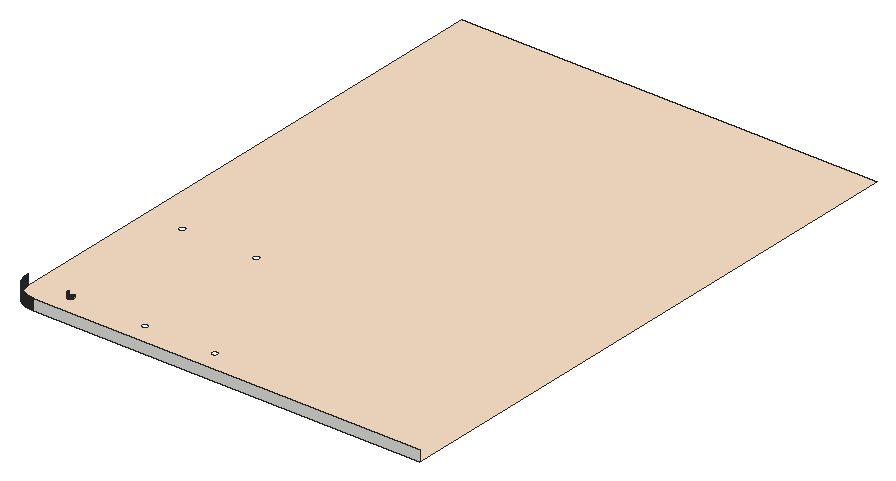
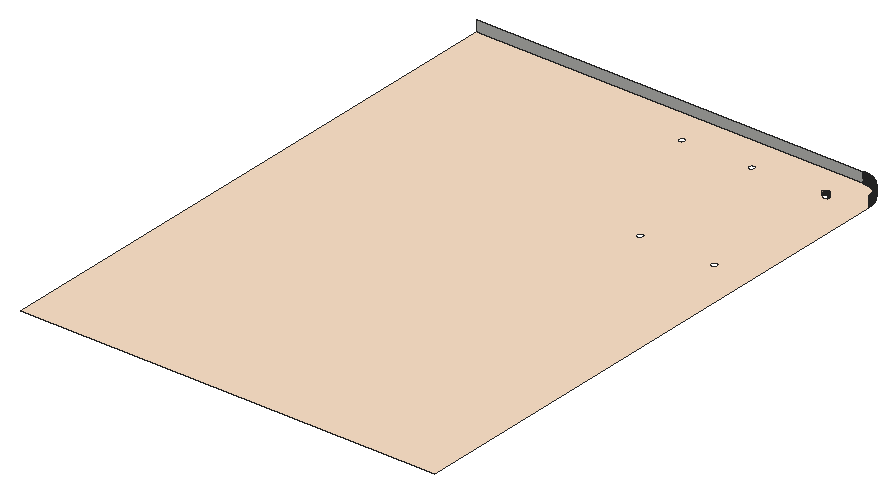
# SketchUp Ruby script. Lengths in inches.
U = 1.inch
M = Sketchup.active_model
def pt(a) = Geom::Point3d.new(a.map { |v| v * U })
def face(e, loops, mat)
  f = e.add_face(loops[0].map { |a| pt(a) })
  loops[1..].each { |l| e.add_face(l.map { |a| pt(a) }).erase! }
  f.material = f.back_material = mat if mat
  f
end
# faces: each face lists its corners as indices into pts; further lists are holes
def faces(e, pts, list, mat = nil) = list.each { |f| face(e, (f[0].is_a?(Array) ? f : [f]).map { |l| l.map { |i| pts[i] } }, mat) }
# xy, xz, yz: faces in a plane at the given z, y or x. An outline is a flat list of corners, or four numbers for a rectangle; further outlines are holes
def ring(l) = l.size == 4 ? [[l[0], l[1]], [l[2], l[1]], [l[2], l[3]], [l[0], l[3]]] : l.each_slice(2).to_a
def flat(e, list, mat, &to3) = list.each { |f| face(e, (f[0].is_a?(Array) ? f : [f]).map { |l| ring(l).map { |u, v| to3.(u, v) } }, mat) }
def xy(e, z, list, mat = nil) = flat(e, list, mat) { |x, y| [x, y, z] }
def xz(e, y, list, mat = nil) = flat(e, list, mat) { |x, z| [x, y, z] }
def yz(e, x, list, mat = nil) = flat(e, list, mat) { |y, z| [x, y, z] }
def lines(e, pts, list) = list.each { |a, b| e.add_line(pt(pts[a]), pt(pts[b])) }
# prism: a flat outline (further loops are holes) pulled along v
def prism(e, loops, v, mat = nil)
  f = face(e, loops, mat); d = Geom::Vector3d.new(v.map { |x| x * U })
  f.pushpull(f.normal.samedirection?(d) ? d.length : -d.length)
end
def box(e, o, s, mat = nil) = prism(e, [[o, [o[0] + s[0], o[1], o[2]], [o[0] + s[0], o[1] + s[1], o[2]], [o[0], o[1] + s[1], o[2]]]], [0, 0, s[2]], mat)
def at(x, y, z, deg = 0) = Geom::Transformation.translation(pt([x, y, z])) * Geom::Transformation.rotation(ORIGIN, Z_AXIS, deg.degrees)
def axes(o, x, y, z) = Geom::Transformation.new([*x, 0, *y, 0, *z, 0, *pt(o).to_a, 1])
def part(name) = M.definitions.add(name)
# library, detail: a bought-in or finely detailed component or shape, given as its bounding box
def library(name, o, s) = part(name).tap { |d| box(d.entities, o, s) }
def detail(e, o, s) = box(e.add_group.entities, o, s)
def put(e, d, t, mat = nil) = e.add_instance(d, t).tap { |i| i.material = mat if mat }
def group(e, t, mat = nil) = e.add_group.tap { |g| g.transformation = t; g.material = mat if mat }.entities
root = M.entities
M.materials.add("1122 AP 7994 PEACH ROSE").color = [254, 227, 201]
xy(root,149.82,[[[32.75,153,32.5,153.01,32.25,153.01,31.99,153.02,31.74,153.03,31.49,153.05,31.24,153.0625,30.99,153.08,30.74,153.11,30.49,153.13,30.24,153.16,29.99,153.1875,29.74,153.22,29.49,153.26,29.25,153.3,28.75,153.38,28.5,153.43,28.26,153.47,28.01,153.52,27.76,153.58,27.52,153.63,27.28,153.69,27.03,153.75,26.79,153.82,26.55,153.88,26.3,153.95,26.0625,154.02,25.82,154.1,25.58,154.17,25.34,154.25,25.11,154.33,24.63,154.51,24.4,154.59,24.17,154.69,23.93,154.78,23.47,154.97,23.24,155.07,23.01,155.18,22.78,155.28,22.55,155.39,22.33,155.5,22.1,155.62,21.88,155.73,21.66,155.85,21.4375,155.97,21.22,156.09,21,156.22,20.78,156.34,20.57,156.47,20.35,156.6,20.14,156.74,19.93,156.87,19.3,157.29,19.1,157.4375,18.89,157.58,18.49,157.88,18.29,158.04,18.09,158.19,17.9,158.35,17.7,158.51,17.32,158.83,17.13,159,16.94,159.16,16.75,159.33,16.57,159.5,16.39,159.68,16.21,159.85,15.85,160.21,15.68,160.39,15.5,160.57,15.33,160.75,15.16,160.94,15,161.13,14.83,161.32,14.51,161.7,14.35,161.9,14.19,162.09,14.04,162.29,13.88,162.49,13.58,162.89,13.4375,163.1,13.29,163.3,12.87,163.93,12.74,164.14,12.6,164.35,12.47,164.57,12.34,164.78,12.22,165,12.09,165.22,11.97,165.4375,11.85,165.66,11.73,165.88,11.62,166.1,11.5,166.33,11.39,166.55,11.28,166.78,11.18,167.01,11.07,167.24,10.97,167.47,10.78,167.93,10.69,168.17,10.59,168.4,10.51,168.63,10.33,169.11,10.25,169.34,10.17,169.58,10.1,169.82,10.02,170.0625,9.95,170.3,9.88,170.55,9.82,170.79,9.75,171.03,9.69,171.28,9.63,171.52,9.58,171.76,9.52,172.01,9.47,172.26,9.43,172.5,9.38,172.75,9.3,173.25,9.26,173.49,9.22,173.74,9.1875,173.99,9.16,174.24,9.13,174.49,9.11,174.74,9.08,174.99,9.0625,175.24,9.05,175.49,9.03,175.74,9.02,175.99,9.01,176.25,9.01,176.5,9,176.75,9,645,366,645,366,153],[40.86,180.07,41.17,180.07,41.49,180.11,41.5625,180.12,41.64,180.14,41.72,180.15,41.79,180.17,41.87,180.19,41.94,180.22,42.02,180.24,42.16,180.3,42.24,180.33,42.31,180.36,42.38,180.4,42.45,180.43,42.52,180.47,42.58,180.51,42.65,180.55,42.72,180.6,42.78,180.64,43.08,180.89,43.14,180.95,43.19,181.01,43.25,181.0625,43.3,181.12,43.4,181.24,43.44,181.31,43.49,181.37,43.53,181.4375,43.57,181.5,43.65,181.64,43.6875,181.71,43.72,181.78,43.76,181.85,43.79,181.92,43.82,182,43.84,182.07,43.87,182.14,43.89,182.22,43.91,182.29,43.95,182.45,43.97,182.52,44.01,182.84,44.01,182.91,44.02,182.99,44.02,183.15,44.01,183.23,44.01,183.31,44,183.38,43.97,183.62,43.95,183.69,43.91,183.85,43.89,183.92,43.87,184,43.84,184.07,43.82,184.15,43.76,184.29,43.72,184.36,43.6875,184.43,43.65,184.5,43.57,184.64,43.53,184.7,43.49,184.77,43.44,184.83,43.4,184.9,43.25,185.08,43.08,185.25,42.78,185.5,42.72,185.54,42.65,185.59,42.58,185.63,42.52,185.67,42.45,185.71,42.38,185.74,42.31,185.78,42.24,185.8125,42.16,185.84,42.02,185.9,41.94,185.92,41.87,185.95,41.79,185.97,41.72,185.99,41.64,186.01,41.5625,186.02,41.49,186.03,41.41,186.05,41.33,186.05,41.25,186.0625,41.17,186.07,40.86,186.07,40.78,186.0625,40.7,186.05,40.625,186.05,40.55,186.03,40.39,186.01,40.32,185.99,40.16,185.95,40.09,185.92,40.01,185.9,39.87,185.84,39.8,185.8125,39.72,185.78,39.65,185.74,39.58,185.71,39.52,185.67,39.38,185.59,39.32,185.54,39.25,185.5,38.95,185.25,38.84,185.14,38.74,185.02,38.68,184.96,38.64,184.9,38.59,184.83,38.54,184.77,38.5,184.7,38.46,184.64,38.34,184.43,38.28,184.29,38.24,184.22,38.22,184.15,38.1875,184.07,38.16,184,38.14,183.92,38.12,183.85,38.08,183.69,38.07,183.62,38.05,183.54,38.03,183.38,38.03,183.31,38.02,183.23,38.02,182.91,38.03,182.84,38.03,182.76,38.05,182.6,38.07,182.52,38.08,182.45,38.12,182.29,38.14,182.22,38.16,182.14,38.1875,182.07,38.22,182,38.24,181.92,38.28,181.85,38.34,181.71,38.46,181.5,38.5,181.4375,38.54,181.37,38.59,181.31,38.64,181.24,38.68,181.18,38.74,181.12,38.79,181.0625,38.84,181.01,38.89,180.95,38.95,180.89,39.25,180.64,39.32,180.6,39.38,180.55,39.52,180.47,39.58,180.43,39.65,180.4,39.72,180.36,39.8,180.33,40.01,180.24,40.09,180.22,40.16,180.19,40.32,180.15,40.39,180.14,40.47,180.12,40.55,180.11,40.7,180.09],[104.79,180.07,105.11,180.07,105.1875,180.08,105.26,180.09,105.5,180.12,105.57,180.14,105.65,180.15,105.73,180.17,105.8,180.19,105.88,180.22,105.95,180.24,106.03,180.27,106.24,180.36,106.3125,180.4,106.38,180.43,106.59,180.55,106.65,180.6,106.71,180.64,106.78,180.69,107.02,180.89,107.07,180.95,107.13,181.01,107.18,181.0625,107.23,181.12,107.33,181.24,107.38,181.31,107.42,181.37,107.47,181.4375,107.51,181.5,107.59,181.64,107.66,181.78,107.72,181.92,107.75,182,107.78,182.07,107.8,182.14,107.83,182.22,107.85,182.29,107.89,182.45,107.9,182.52,107.91,182.6,107.93,182.68,107.93,182.76,107.94,182.84,107.95,182.91,107.95,183.23,107.94,183.31,107.93,183.38,107.93,183.46,107.91,183.54,107.9,183.62,107.89,183.69,107.85,183.85,107.83,183.92,107.8,184,107.78,184.07,107.75,184.15,107.66,184.36,107.59,184.5,107.51,184.64,107.47,184.7,107.42,184.77,107.38,184.83,107.33,184.9,107.13,185.14,107.07,185.19,107.02,185.25,106.78,185.45,106.71,185.5,106.65,185.54,106.59,185.59,106.38,185.71,106.3125,185.74,106.24,185.78,106.17,185.8125,106.1,185.84,106.03,185.87,105.95,185.9,105.88,185.92,105.8,185.95,105.73,185.97,105.57,186.01,105.5,186.02,105.42,186.03,105.34,186.05,105.26,186.05,105.1875,186.0625,105.11,186.07,104.79,186.07,104.72,186.0625,104.64,186.05,104.56,186.05,104.48,186.03,104.4,186.02,104.33,186.01,104.17,185.97,104.1,185.95,104.02,185.92,103.95,185.9,103.8,185.84,103.73,185.8125,103.66,185.78,103.59,185.74,103.52,185.71,103.38,185.63,103.32,185.59,103.25,185.54,103.1875,185.5,103,185.35,102.94,185.3,102.72,185.08,102.57,184.9,102.52,184.83,102.48,184.77,102.44,184.7,102.39,184.64,102.31,184.5,102.28,184.43,102.24,184.36,102.15,184.15,102.125,184.07,102.1,184,102.07,183.92,102.05,183.85,102.03,183.77,102.02,183.69,102,183.62,101.97,183.38,101.96,183.31,101.96,183.23,101.95,183.15,101.95,182.99,101.96,182.91,101.96,182.84,102,182.52,102.02,182.45,102.03,182.37,102.05,182.29,102.07,182.22,102.1,182.14,102.15,182,102.18,181.92,102.24,181.78,102.28,181.71,102.31,181.64,102.39,181.5,102.44,181.4375,102.48,181.37,102.52,181.31,102.57,181.24,102.67,181.12,102.72,181.0625,102.78,181.01,102.83,180.95,102.94,180.84,103,180.79,103.1875,180.64,103.25,180.6,103.32,180.55,103.38,180.51,103.52,180.43,103.59,180.4,103.66,180.36,103.8,180.3,103.95,180.24,104.02,180.22,104.1,180.19,104.17,180.17,104.25,180.15,104.33,180.14,104.4,180.12,104.72,180.08],[164.79,180.07,165.11,180.07,165.1875,180.08,165.26,180.09,165.5,180.12,165.57,180.14,165.65,180.15,165.73,180.17,165.8,180.19,165.88,180.22,165.95,180.24,166.03,180.27,166.24,180.36,166.3125,180.4,166.38,180.43,166.59,180.55,166.65,180.6,166.71,180.64,166.78,180.69,167.02,180.89,167.07,180.95,167.13,181.01,167.18,181.0625,167.23,181.12,167.33,181.24,167.38,181.31,167.42,181.37,167.47,181.4375,167.51,181.5,167.59,181.64,167.66,181.78,167.72,181.92,167.75,182,167.78,182.07,167.8,182.14,167.83,182.22,167.85,182.29,167.89,182.45,167.9,182.52,167.91,182.6,167.93,182.68,167.93,182.76,167.94,182.84,167.95,182.91,167.95,183.23,167.94,183.31,167.93,183.38,167.93,183.46,167.91,183.54,167.9,183.62,167.89,183.69,167.85,183.85,167.83,183.92,167.8,184,167.78,184.07,167.75,184.15,167.66,184.36,167.59,184.5,167.51,184.64,167.47,184.7,167.42,184.77,167.38,184.83,167.33,184.9,167.13,185.14,167.07,185.19,167.02,185.25,166.78,185.45,166.71,185.5,166.65,185.54,166.59,185.59,166.38,185.71,166.3125,185.74,166.24,185.78,166.17,185.8125,166.1,185.84,166.03,185.87,165.95,185.9,165.88,185.92,165.8,185.95,165.73,185.97,165.57,186.01,165.5,186.02,165.42,186.03,165.34,186.05,165.26,186.05,165.1875,186.0625,165.11,186.07,164.79,186.07,164.72,186.0625,164.64,186.05,164.56,186.05,164.48,186.03,164.4,186.02,164.33,186.01,164.17,185.97,164.1,185.95,164.02,185.92,163.95,185.9,163.8,185.84,163.73,185.8125,163.66,185.78,163.59,185.74,163.52,185.71,163.38,185.63,163.32,185.59,163.25,185.54,163.1875,185.5,163,185.35,162.94,185.3,162.72,185.08,162.57,184.9,162.52,184.83,162.48,184.77,162.44,184.7,162.39,184.64,162.31,184.5,162.28,184.43,162.24,184.36,162.15,184.15,162.125,184.07,162.1,184,162.07,183.92,162.05,183.85,162.03,183.77,162.02,183.69,162,183.62,161.97,183.38,161.96,183.31,161.96,183.23,161.95,183.15,161.95,182.99,161.96,182.91,161.96,182.84,162,182.52,162.02,182.45,162.03,182.37,162.05,182.29,162.07,182.22,162.1,182.14,162.15,182,162.18,181.92,162.24,181.78,162.28,181.71,162.31,181.64,162.39,181.5,162.44,181.4375,162.48,181.37,162.52,181.31,162.57,181.24,162.67,181.12,162.72,181.0625,162.78,181.01,162.83,180.95,162.94,180.84,163,180.79,163.1875,180.64,163.25,180.6,163.32,180.55,163.38,180.51,163.52,180.43,163.59,180.4,163.66,180.36,163.8,180.3,163.95,180.24,164.02,180.22,164.1,180.19,164.17,180.17,164.25,180.15,164.33,180.14,164.4,180.12,164.72,180.08],[104.79,300.07,105.11,300.07,105.1875,300.08,105.26,300.09,105.5,300.12,105.57,300.14,105.65,300.15,105.73,300.17,105.8,300.19,105.88,300.22,105.95,300.24,106.03,300.27,106.24,300.36,106.3125,300.4,106.38,300.43,106.59,300.55,106.65,300.6,106.71,300.64,106.78,300.69,107.02,300.89,107.07,300.95,107.13,301.01,107.18,301.0625,107.23,301.12,107.33,301.24,107.38,301.31,107.42,301.37,107.47,301.4375,107.51,301.5,107.59,301.64,107.66,301.78,107.72,301.92,107.75,302,107.78,302.07,107.8,302.14,107.83,302.22,107.85,302.29,107.89,302.45,107.9,302.52,107.91,302.6,107.93,302.68,107.93,302.76,107.94,302.84,107.95,302.91,107.95,303.23,107.94,303.31,107.93,303.38,107.93,303.46,107.91,303.54,107.9,303.62,107.89,303.69,107.85,303.85,107.83,303.92,107.8,304,107.78,304.07,107.75,304.15,107.66,304.36,107.59,304.5,107.51,304.64,107.47,304.7,107.42,304.77,107.38,304.83,107.33,304.9,107.13,305.14,107.07,305.19,107.02,305.25,106.78,305.45,106.71,305.5,106.65,305.54,106.59,305.59,106.38,305.71,106.3125,305.74,106.24,305.78,106.17,305.8125,106.1,305.84,106.03,305.87,105.95,305.9,105.88,305.92,105.8,305.95,105.73,305.97,105.57,306.01,105.5,306.02,105.42,306.03,105.34,306.05,105.26,306.05,105.1875,306.0625,105.11,306.07,104.79,306.07,104.72,306.0625,104.64,306.05,104.56,306.05,104.48,306.03,104.4,306.02,104.33,306.01,104.17,305.97,104.1,305.95,104.02,305.92,103.95,305.9,103.8,305.84,103.73,305.8125,103.66,305.78,103.59,305.74,103.52,305.71,103.38,305.63,103.32,305.59,103.25,305.54,103.1875,305.5,103,305.35,102.94,305.3,102.72,305.08,102.57,304.9,102.52,304.83,102.48,304.77,102.44,304.7,102.39,304.64,102.31,304.5,102.28,304.43,102.24,304.36,102.15,304.15,102.125,304.07,102.1,304,102.07,303.92,102.05,303.85,102.03,303.77,102.02,303.69,102,303.62,101.97,303.38,101.96,303.31,101.96,303.23,101.95,303.15,101.95,302.99,101.96,302.91,101.96,302.84,102,302.52,102.02,302.45,102.03,302.37,102.05,302.29,102.07,302.22,102.1,302.14,102.15,302,102.18,301.92,102.24,301.78,102.28,301.71,102.31,301.64,102.39,301.5,102.44,301.4375,102.48,301.37,102.52,301.31,102.57,301.24,102.67,301.12,102.72,301.0625,102.78,301.01,102.83,300.95,102.94,300.84,103,300.79,103.1875,300.64,103.25,300.6,103.32,300.55,103.38,300.51,103.52,300.43,103.59,300.4,103.66,300.36,103.8,300.3,103.95,300.24,104.02,300.22,104.1,300.19,104.17,300.17,104.25,300.15,104.33,300.14,104.4,300.12,104.72,300.08],[40.86,300.07,41.17,300.07,41.49,300.11,41.5625,300.12,41.64,300.14,41.72,300.15,41.79,300.17,41.87,300.19,41.94,300.22,42.02,300.24,42.16,300.3,42.24,300.33,42.31,300.36,42.38,300.4,42.45,300.43,42.52,300.47,42.58,300.51,42.65,300.55,42.72,300.6,42.78,300.64,43.08,300.89,43.14,300.95,43.19,301.01,43.25,301.0625,43.3,301.12,43.4,301.24,43.44,301.31,43.49,301.37,43.53,301.4375,43.57,301.5,43.65,301.64,43.6875,301.71,43.72,301.78,43.76,301.85,43.79,301.92,43.82,302,43.84,302.07,43.87,302.14,43.89,302.22,43.91,302.29,43.95,302.45,43.97,302.52,44.01,302.84,44.01,302.91,44.02,302.99,44.02,303.15,44.01,303.23,44.01,303.31,44,303.38,43.97,303.62,43.95,303.69,43.91,303.85,43.89,303.92,43.87,304,43.84,304.07,43.82,304.15,43.76,304.29,43.72,304.36,43.6875,304.43,43.65,304.5,43.57,304.64,43.53,304.7,43.49,304.77,43.44,304.83,43.4,304.9,43.25,305.08,43.08,305.25,42.78,305.5,42.72,305.54,42.65,305.59,42.58,305.63,42.52,305.67,42.45,305.71,42.38,305.74,42.31,305.78,42.24,305.8125,42.16,305.84,42.02,305.9,41.94,305.92,41.87,305.95,41.79,305.97,41.72,305.99,41.64,306.01,41.5625,306.02,41.49,306.03,41.41,306.05,41.33,306.05,41.25,306.0625,41.17,306.07,40.86,306.07,40.78,306.0625,40.7,306.05,40.625,306.05,40.55,306.03,40.39,306.01,40.32,305.99,40.16,305.95,40.09,305.92,40.01,305.9,39.87,305.84,39.8,305.8125,39.72,305.78,39.65,305.74,39.58,305.71,39.52,305.67,39.38,305.59,39.32,305.54,39.25,305.5,38.95,305.25,38.84,305.14,38.74,305.02,38.68,304.96,38.64,304.9,38.59,304.83,38.54,304.77,38.5,304.7,38.46,304.64,38.34,304.43,38.28,304.29,38.24,304.22,38.22,304.15,38.1875,304.07,38.16,304,38.14,303.92,38.12,303.85,38.08,303.69,38.07,303.62,38.05,303.54,38.03,303.38,38.03,303.31,38.02,303.23,38.02,302.91,38.03,302.84,38.03,302.76,38.05,302.6,38.07,302.52,38.08,302.45,38.12,302.29,38.14,302.22,38.16,302.14,38.1875,302.07,38.22,302,38.24,301.92,38.28,301.85,38.34,301.71,38.46,301.5,38.5,301.4375,38.54,301.37,38.59,301.31,38.64,301.24,38.68,301.18,38.74,301.12,38.79,301.0625,38.84,301.01,38.89,300.95,38.95,300.89,39.25,300.64,39.32,300.6,39.38,300.55,39.52,300.47,39.58,300.43,39.65,300.4,39.72,300.36,39.8,300.33,40.01,300.24,40.09,300.22,40.16,300.19,40.32,300.15,40.39,300.14,40.47,300.12,40.55,300.11,40.7,300.09]]],"1122 AP 7994 PEACH ROSE")
xz(root,153,[[32.75,149.82,33,158.82],[33,149.82,366,158.82]])
xz(root,153.01,[[32.25,149.82,32.5,158.82]])
xz(root,180.07,[[40.86,149.82,40.9375,152.82],[40.9375,149.82,41.02,152.82],[41.02,149.82,41.09,152.82],[41.09,149.82,41.17,152.82]],"1122 AP 7994 PEACH ROSE")
yz(root,9,[[176.75,149.82,177,158.82]])
yz(root,9.01,[[176.25,149.82,176.5,158.82]])
yz(root,38.02,[[182.91,149.82,182.99,152.82],[182.99,149.82,183.07,152.82],[183.07,149.82,183.15,152.82],[183.15,149.82,183.23,152.82]],"1122 AP 7994 PEACH ROSE")
yz(root,38.03,[[182.76,149.82,182.84,152.82],[183.31,149.82,183.38,152.82]],"1122 AP 7994 PEACH ROSE")
yz(root,44.01,[[182.84,149.82,182.91,152.82]],"1122 AP 7994 PEACH ROSE")
yz(root,44.02,[[182.99,149.82,183.07,152.82]],"1122 AP 7994 PEACH ROSE")
p = [[31.49,153.05,158.82],[31.24,153.0625,158.82],[31.24,153.0625,149.82],[31.49,153.05,149.82],[31.74,153.03,158.82],[31.74,153.03,149.82],
  [31.99,153.02,158.82],[31.99,153.02,149.82],[32.25,153.01,158.82],[32.25,153.01,149.82],[32.75,153,158.82],[32.5,153.01,158.82],
  [32.5,153.01,149.82],[32.75,153,149.82],[30.49,153.13,158.82],[30.24,153.16,158.82],[30.24,153.16,149.82],[30.49,153.13,149.82],
  [30.74,153.11,158.82],[30.74,153.11,149.82],[30.99,153.08,158.82],[30.99,153.08,149.82],[29.74,153.22,158.82],[29.49,153.26,158.82],
  [29.49,153.26,149.82],[29.74,153.22,149.82],[29.99,153.1875,158.82],[29.99,153.1875,149.82],[29,153.34,158.82],[28.75,153.38,158.82],
  [28.75,153.38,149.82],[29,153.34,149.82],[29.25,153.3,158.82],[29.25,153.3,149.82],[28.5,153.43,158.82],[28.26,153.47,158.82],
  [28.26,153.47,149.82],[28.5,153.43,149.82],[28.01,153.52,158.82],[27.76,153.58,158.82],[27.76,153.58,149.82],[28.01,153.52,149.82],
  [27.52,153.63,158.82],[27.28,153.69,158.82],[27.28,153.69,149.82],[27.52,153.63,149.82],[27.03,153.75,158.82],[27.03,153.75,149.82],
  [26.79,153.82,158.82],[26.55,153.88,158.82],[26.55,153.88,149.82],[26.79,153.82,149.82],[26.3,153.95,158.82],[26.3,153.95,149.82],
  [26.0625,154.02,158.82],[25.82,154.1,158.82],[25.82,154.1,149.82],[26.0625,154.02,149.82],[25.58,154.17,158.82],[25.58,154.17,149.82],
  [25.34,154.25,158.82],[25.34,154.25,149.82],[25.11,154.33,158.82],[24.87,154.42,158.82],[24.87,154.42,149.82],[25.11,154.33,149.82],
  [24.63,154.51,158.82],[24.63,154.51,149.82],[24.4,154.59,158.82],[24.4,154.59,149.82],[24.17,154.69,158.82],[24.17,154.69,149.82],
  [23.93,154.78,158.82],[23.93,154.78,149.82],[23.7,154.875,158.82],[23.7,154.875,149.82],[23.47,154.97,158.82],[23.47,154.97,149.82],
  [23.24,155.07,158.82],[23.24,155.07,149.82],[23.01,155.18,158.82],[23.01,155.18,149.82],[22.78,155.28,158.82],[22.78,155.28,149.82],
  [22.55,155.39,158.82],[22.55,155.39,149.82],[22.33,155.5,158.82],[22.33,155.5,149.82],[22.1,155.62,158.82],[22.1,155.62,149.82],
  [21.88,155.73,158.82],[21.88,155.73,149.82],[21.66,155.85,158.82],[21.66,155.85,149.82],[21.4375,155.97,158.82],[21.4375,155.97,149.82],
  [21.22,156.09,158.82],[21.22,156.09,149.82],[21,156.22,158.82],[21,156.22,149.82],[20.78,156.34,158.82],[20.78,156.34,149.82],
  [20.57,156.47,158.82],[20.57,156.47,149.82],[20.35,156.6,158.82],[20.35,156.6,149.82],[20.14,156.74,158.82],[20.14,156.74,149.82],
  [19.93,156.87,158.82],[19.93,156.87,149.82],[19.72,157.01,158.82],[19.72,157.01,149.82],[19.51,157.15,158.82],[19.51,157.15,149.82],
  [19.3,157.29,158.82],[19.3,157.29,149.82],[19.1,157.4375,158.82],[19.1,157.4375,149.82],[18.89,157.58,158.82],[18.89,157.58,149.82],
  [18.69,157.73,158.82],[18.69,157.73,149.82],[18.49,157.88,158.82],[18.49,157.88,149.82],[18.29,158.04,158.82],[18.29,158.04,149.82],
  [18.09,158.19,158.82],[18.09,158.19,149.82],[17.9,158.35,158.82],[17.9,158.35,149.82],[17.7,158.51,158.82],[17.7,158.51,149.82],
  [17.51,158.67,158.82],[17.51,158.67,149.82],[17.32,158.83,158.82],[17.32,158.83,149.82],[17.13,159,158.82],[17.13,159,149.82],
  [16.94,159.16,158.82],[16.94,159.16,149.82],[16.75,159.33,158.82],[16.75,159.33,149.82],[16.57,159.5,158.82],[16.57,159.5,149.82],
  [16.39,159.68,158.82],[16.39,159.68,149.82],[16.21,159.85,158.82],[16.21,159.85,149.82],[16.03,160.03,158.82],[16.03,160.03,149.82],
  [15.85,160.21,158.82],[15.85,160.21,149.82],[15.68,160.39,158.82],[15.68,160.39,149.82],[15.5,160.57,158.82],[15.5,160.57,149.82],
  [15.33,160.75,158.82],[15.33,160.75,149.82],[15.16,160.94,158.82],[15.16,160.94,149.82],[15,161.13,158.82],[15,161.13,149.82],
  [14.83,161.32,158.82],[14.83,161.32,149.82],[14.67,161.51,158.82],[14.67,161.51,149.82],[14.51,161.7,158.82],[14.51,161.7,149.82],
  [14.35,161.9,158.82],[14.35,161.9,149.82],[14.19,162.09,158.82],[14.19,162.09,149.82],[14.04,162.29,158.82],[14.04,162.29,149.82],
  [13.88,162.49,158.82],[13.88,162.49,149.82],[13.73,162.69,158.82],[13.73,162.69,149.82],[13.58,162.89,158.82],[13.58,162.89,149.82],
  [13.4375,163.1,158.82],[13.4375,163.1,149.82],[13.29,163.3,158.82],[13.29,163.3,149.82],[13.15,163.51,158.82],[13.15,163.51,149.82],
  [13.01,163.72,158.82],[13.01,163.72,149.82],[12.87,163.93,158.82],[12.87,163.93,149.82],[12.74,164.14,158.82],[12.74,164.14,149.82],
  [12.6,164.35,158.82],[12.6,164.35,149.82],[12.47,164.57,158.82],[12.47,164.57,149.82],[12.34,164.78,158.82],[12.34,164.78,149.82],
  [12.22,165,158.82],[12.22,165,149.82],[12.09,165.22,158.82],[12.09,165.22,149.82],[11.97,165.4375,158.82],[11.97,165.4375,149.82],
  [11.85,165.66,158.82],[11.85,165.66,149.82],[11.73,165.88,158.82],[11.73,165.88,149.82],[11.62,166.1,158.82],[11.62,166.1,149.82],
  [11.5,166.33,158.82],[11.5,166.33,149.82],[11.39,166.55,158.82],[11.39,166.55,149.82],[11.28,166.78,158.82],[11.28,166.78,149.82],
  [11.18,167.01,158.82],[11.18,167.01,149.82],[11.07,167.24,158.82],[11.07,167.24,149.82],[10.97,167.47,158.82],[10.97,167.47,149.82],
  [10.875,167.7,158.82],[10.875,167.7,149.82],[10.78,167.93,158.82],[10.78,167.93,149.82],[10.69,168.17,158.82],[10.69,168.17,149.82],
  [10.59,168.4,158.82],[10.59,168.4,149.82],[10.51,168.63,158.82],[10.51,168.63,149.82],[10.42,168.87,158.82],[10.42,168.87,149.82],
  [10.33,169.11,158.82],[10.33,169.11,149.82],[10.25,169.34,158.82],[10.25,169.34,149.82],[10.17,169.58,158.82],[10.17,169.58,149.82],
  [10.1,169.82,158.82],[10.1,169.82,149.82],[10.02,170.0625,158.82],[10.02,170.0625,149.82],[9.95,170.3,158.82],[9.95,170.3,149.82],
  [9.88,170.55,158.82],[9.88,170.55,149.82],[9.82,170.79,158.82],[9.82,170.79,149.82],[9.75,171.03,158.82],[9.75,171.03,149.82],
  [9.69,171.28,158.82],[9.69,171.28,149.82],[9.63,171.52,158.82],[9.63,171.52,149.82],[9.58,171.76,158.82],[9.58,171.76,149.82],
  [9.52,172.01,158.82],[9.52,172.01,149.82],[9.47,172.26,158.82],[9.47,172.26,149.82],[9.43,172.5,158.82],[9.43,172.5,149.82],
  [9.38,172.75,158.82],[9.38,172.75,149.82],[9.34,173,158.82],[9.34,173,149.82],[9.3,173.25,158.82],[9.3,173.25,149.82],
  [9.26,173.49,158.82],[9.26,173.49,149.82],[9.22,173.74,158.82],[9.22,173.74,149.82],[9.1875,173.99,158.82],[9.1875,173.99,149.82],
  [9.16,174.24,158.82],[9.16,174.24,149.82],[9.13,174.49,158.82],[9.13,174.49,149.82],[9.11,174.74,158.82],[9.11,174.74,149.82],
  [9.08,174.99,158.82],[9.08,174.99,149.82],[9.0625,175.24,158.82],[9.0625,175.24,149.82],[9.05,175.49,158.82],[9.05,175.49,149.82],
  [9.03,175.74,158.82],[9.03,175.74,149.82],[9.02,175.99,158.82],[9.02,175.99,149.82],[9.01,176.25,158.82],[9.01,176.25,149.82],
  [9.01,176.5,158.82],[9,176.75,158.82],[9,176.75,149.82],[9.01,176.5,149.82],[40.39,180.14,149.82],[40.32,180.15,149.82],
  [40.32,180.15,152.82],[40.39,180.14,152.82],[40.47,180.12,149.82],[40.47,180.12,152.82],[40.625,180.1,149.82],[40.55,180.11,149.82],
  [40.55,180.11,152.82],[40.625,180.1,152.82],[40.7,180.09,149.82],[40.7,180.09,152.82],[40.78,180.08,149.82],[40.78,180.08,152.82],
  [40.86,180.07,149.82],[40.86,180.07,152.82],[41.25,180.08,149.82],[41.17,180.07,149.82],[41.17,180.07,152.82],[41.25,180.08,152.82],
  [41.33,180.09,149.82],[41.33,180.09,152.82],[41.41,180.1,149.82],[41.41,180.1,152.82],[41.49,180.11,149.82],[41.49,180.11,152.82],
  [41.5625,180.12,149.82],[41.5625,180.12,152.82],[41.64,180.14,149.82],[41.64,180.14,152.82],[41.72,180.15,149.82],[41.72,180.15,152.82],
  [40.01,180.24,149.82],[39.94,180.27,149.82],[39.94,180.27,152.82],[40.01,180.24,152.82],[40.09,180.22,149.82],[40.09,180.22,152.82],
  [40.16,180.19,149.82],[40.16,180.19,152.82],[40.24,180.17,149.82],[40.24,180.17,152.82],[41.79,180.17,149.82],[41.79,180.17,152.82],
  [41.87,180.19,149.82],[41.87,180.19,152.82],[41.94,180.22,149.82],[41.94,180.22,152.82],[42.02,180.24,149.82],[42.02,180.24,152.82],
  [42.09,180.27,149.82],[42.09,180.27,152.82],[39.8,180.33,149.82],[39.72,180.36,149.82],[39.72,180.36,152.82],[39.8,180.33,152.82],
  [39.87,180.3,149.82],[39.87,180.3,152.82],[42.16,180.3,149.82],[42.16,180.3,152.82],[42.24,180.33,149.82],[42.24,180.33,152.82],
  [42.31,180.36,149.82],[42.31,180.36,152.82],[39.58,180.43,149.82],[39.52,180.47,149.82],[39.52,180.47,152.82],[39.58,180.43,152.82],
  [39.65,180.4,149.82],[39.65,180.4,152.82],[42.38,180.4,149.82],[42.38,180.4,152.82],[42.45,180.43,149.82],[42.45,180.43,152.82],
  [42.52,180.47,149.82],[42.52,180.47,152.82],[39.45,180.51,149.82],[39.45,180.51,152.82],[39.38,180.55,149.82],[39.38,180.55,152.82],
  [42.58,180.51,149.82],[42.58,180.51,152.82],[42.65,180.55,149.82],[42.65,180.55,152.82],[39.25,180.64,149.82],[39.19,180.69,149.82],
  [39.19,180.69,152.82],[39.25,180.64,152.82],[39.32,180.6,149.82],[39.32,180.6,152.82],[42.72,180.6,149.82],[42.72,180.6,152.82],
  [42.78,180.64,149.82],[42.78,180.64,152.82],[42.84,180.69,149.82],[42.84,180.69,152.82],[39.13,180.74,149.82],[39.13,180.74,152.82],
  [39.07,180.79,149.82],[39.07,180.79,152.82],[42.9,180.74,149.82],[42.9,180.74,152.82],[42.96,180.79,149.82],[42.96,180.79,152.82],
  [39.01,180.84,149.82],[39.01,180.84,152.82],[38.95,180.89,149.82],[38.95,180.89,152.82],[43.02,180.84,149.82],[43.02,180.84,152.82],
  [43.08,180.89,149.82],[43.08,180.89,152.82],[38.89,180.95,149.82],[38.84,181.01,149.82],[38.84,181.01,152.82],[38.89,180.95,152.82],
  [43.14,180.95,149.82],[43.14,180.95,152.82],[43.19,181.01,149.82],[43.19,181.01,152.82],[38.79,181.0625,149.82],[38.79,181.0625,152.82],
  [43.25,181.0625,149.82],[43.25,181.0625,152.82],[38.74,181.12,149.82],[38.74,181.12,152.82],[38.68,181.18,149.82],[38.68,181.18,152.82],
  [43.3,181.12,149.82],[43.3,181.12,152.82],[43.35,181.18,149.82],[43.35,181.18,152.82],[38.64,181.24,149.82],[38.64,181.24,152.82],
  [38.59,181.31,149.82],[38.59,181.31,152.82],[43.4,181.24,149.82],[43.4,181.24,152.82],[43.44,181.31,149.82],[43.44,181.31,152.82],
  [38.54,181.37,149.82],[38.54,181.37,152.82],[43.49,181.37,149.82],[43.49,181.37,152.82],[38.5,181.4375,149.82],[38.5,181.4375,152.82],
  [38.46,181.5,149.82],[38.46,181.5,152.82],[43.53,181.4375,149.82],[43.53,181.4375,152.82],[43.57,181.5,149.82],[43.57,181.5,152.82],
  [38.42,181.57,149.82],[38.42,181.57,152.82],[43.61,181.57,149.82],[43.61,181.57,152.82],[38.38,181.64,149.82],[38.34,181.71,149.82],
  [38.34,181.71,152.82],[38.38,181.64,152.82],[43.65,181.64,149.82],[43.65,181.64,152.82],[43.6875,181.71,149.82],[43.6875,181.71,152.82],
  [38.31,181.78,149.82],[38.31,181.78,152.82],[43.72,181.78,149.82],[43.72,181.78,152.82],[38.28,181.85,149.82],[38.28,181.85,152.82],
  [43.76,181.85,149.82],[43.76,181.85,152.82],[38.24,181.92,149.82],[38.24,181.92,152.82],[38.22,182,149.82],[38.22,182,152.82],
  [43.79,181.92,149.82],[43.79,181.92,152.82],[43.82,182,149.82],[43.82,182,152.82],[38.1875,182.07,149.82],[38.1875,182.07,152.82],
  [43.84,182.07,149.82],[43.84,182.07,152.82],[38.16,182.14,149.82],[38.14,182.22,149.82],[38.14,182.22,152.82],[38.16,182.14,152.82],
  [43.87,182.14,149.82],[43.87,182.14,152.82],[43.89,182.22,149.82],[43.89,182.22,152.82],[38.12,182.29,149.82],[38.12,182.29,152.82],
  [43.91,182.29,149.82],[43.91,182.29,152.82],[38.1,182.37,149.82],[38.1,182.37,152.82],[43.93,182.37,149.82],[43.93,182.37,152.82],
  [38.08,182.45,149.82],[38.08,182.45,152.82],[38.07,182.52,149.82],[38.07,182.52,152.82],[43.95,182.45,149.82],[43.95,182.45,152.82],
  [43.97,182.52,149.82],[43.97,182.52,152.82],[38.05,182.6,149.82],[38.05,182.6,152.82],[43.98,182.6,149.82],[43.98,182.6,152.82],
  [38.04,182.68,149.82],[38.04,182.68,152.82],[43.99,182.68,149.82],[43.99,182.68,152.82],[38.03,182.76,149.82],[38.03,182.76,152.82],
  [44,182.76,149.82],[44,182.76,152.82],[38.03,182.84,149.82],[38.02,182.91,149.82],[38.02,182.91,152.82],[38.03,182.84,152.82],
  [44.01,182.84,149.82],[44.01,182.84,152.82],[44.02,182.99,149.82],[44.01,182.91,149.82],[44.01,182.91,152.82],[44.02,182.99,152.82],
  [38.02,183.23,149.82],[38.03,183.31,149.82],[38.03,183.31,152.82],[38.02,183.23,152.82],[38.03,183.38,149.82],[38.04,183.46,149.82],
  [38.04,183.46,152.82],[38.03,183.38,152.82],[38.05,183.54,149.82],[38.05,183.54,152.82],[38.07,183.62,149.82],[38.07,183.62,152.82],
  [38.08,183.69,149.82],[38.08,183.69,152.82],[38.1,183.77,149.82],[38.1,183.77,152.82],[38.12,183.85,149.82],[38.12,183.85,152.82],
  [38.14,183.92,149.82],[38.14,183.92,152.82],[38.16,184,149.82],[38.16,184,152.82],[38.1875,184.07,149.82],[38.1875,184.07,152.82],
  [38.22,184.15,149.82],[38.22,184.15,152.82],[38.24,184.22,149.82],[38.24,184.22,152.82],[38.28,184.29,149.82],[38.28,184.29,152.82],
  [38.31,184.36,149.82],[38.31,184.36,152.82],[38.34,184.43,149.82],[38.34,184.43,152.82],[38.38,184.5,149.82],[38.38,184.5,152.82]]
faces(root,p,[[0,1,2,3],[4,0,3,5],[6,4,5,7],[8,6,7,9],[10,11,12,13],[14,15,16,17],[18,14,17,19],[20,18,19,21],
  [1,20,21,2],[22,23,24,25],[26,22,25,27],[15,26,27,16],[28,29,30,31],[32,28,31,33],[23,32,33,24],[34,35,36,37],
  [29,34,37,30],[38,39,40,41],[35,38,41,36],[42,43,44,45],[39,42,45,40],[43,46,47,44],[48,49,50,51],[46,48,51,47],
  [49,52,53,50],[54,55,56,57],[52,54,57,53],[55,58,59,56],[58,60,61,59],[62,63,64,65],[60,62,65,61],[63,66,67,64],
  [66,68,69,67],[68,70,71,69],[70,72,73,71],[72,74,75,73],[74,76,77,75],[76,78,79,77],[78,80,81,79],[80,82,83,81],
  [82,84,85,83],[84,86,87,85],[86,88,89,87],[88,90,91,89],[90,92,93,91],[92,94,95,93],[94,96,97,95],[96,98,99,97],
  [98,100,101,99],[100,102,103,101],[102,104,105,103],[104,106,107,105],[106,108,109,107],[108,110,111,109],[110,112,113,111],[112,114,115,113],
  [114,116,117,115],[116,118,119,117],[118,120,121,119],[120,122,123,121],[122,124,125,123],[124,126,127,125],[126,128,129,127],[128,130,131,129],
  [130,132,133,131],[132,134,135,133],[134,136,137,135],[136,138,139,137],[138,140,141,139],[140,142,143,141],[142,144,145,143],[144,146,147,145],
  [146,148,149,147],[148,150,151,149],[150,152,153,151],[152,154,155,153],[154,156,157,155],[156,158,159,157],[158,160,161,159],[160,162,163,161],
  [162,164,165,163],[164,166,167,165],[166,168,169,167],[168,170,171,169],[170,172,173,171],[172,174,175,173],[174,176,177,175],[176,178,179,177],
  [178,180,181,179],[180,182,183,181],[182,184,185,183],[184,186,187,185],[186,188,189,187],[188,190,191,189],[190,192,193,191],[192,194,195,193],
  [194,196,197,195],[196,198,199,197],[198,200,201,199],[200,202,203,201],[202,204,205,203],[204,206,207,205],[206,208,209,207],[208,210,211,209],
  [210,212,213,211],[212,214,215,213],[214,216,217,215],[216,218,219,217],[218,220,221,219],[220,222,223,221],[222,224,225,223],[224,226,227,225],
  [226,228,229,227],[228,230,231,229],[230,232,233,231],[232,234,235,233],[234,236,237,235],[236,238,239,237],[238,240,241,239],[240,242,243,241],
  [242,244,245,243],[244,246,247,245],[246,248,249,247],[248,250,251,249],[250,252,253,251],[252,254,255,253],[254,256,257,255],[256,258,259,257],
  [258,260,261,259],[260,262,263,261],[262,264,265,263],[264,266,267,265],[266,268,269,267],[268,270,271,269],[270,272,273,271],[272,274,275,273],
  [274,276,277,275],[276,278,279,277],[278,280,281,279],[280,282,283,281],[282,284,285,283],[284,286,287,285],[286,288,289,287],[288,290,291,289],
  [290,292,293,291],[294,295,296,297]])
faces(root,p,[[298,299,300,301],[302,298,301,303],[304,305,306,307],[305,302,303,306],[308,304,307,309],[310,308,309,311],[312,310,311,313],[314,315,316,317],
  [318,314,317,319],[320,318,319,321],[322,320,321,323],[324,322,323,325],[326,324,325,327],[328,326,327,329],[330,331,332,333],[334,330,333,335],
  [336,334,335,337],[299,338,339,300],[338,336,337,339],[340,328,329,341],[342,340,341,343],[344,342,343,345],[346,344,345,347],[348,346,347,349],
  [350,351,352,353],[354,350,353,355],[331,354,355,332],[356,348,349,357],[358,356,357,359],[360,358,359,361],[362,363,364,365],[366,362,365,367],
  [351,366,367,352],[368,360,361,369],[370,368,369,371],[372,370,371,373],[363,374,375,364],[374,376,377,375],[378,372,373,379],[380,378,379,381],
  [382,383,384,385],[376,386,387,377],[386,382,385,387],[388,380,381,389],[390,388,389,391],[392,390,391,393],[383,394,395,384],[394,396,397,395],
  [398,392,393,399],[400,398,399,401],[396,402,403,397],[402,404,405,403],[406,400,401,407],[408,406,407,409],[410,411,412,413],[404,410,413,405],
  [414,408,409,415],[416,414,415,417],[411,418,419,412],[420,416,417,421],[418,422,423,419],[422,424,425,423],[426,420,421,427],[428,426,427,429],
  [424,430,431,425],[430,432,433,431],[434,428,429,435],[436,434,435,437],[432,438,439,433],[440,436,437,441],[438,442,443,439],[442,444,445,443],
  [446,440,441,447],[448,446,447,449],[444,450,451,445],[452,448,449,453],[454,455,456,457],[450,454,457,451],[458,452,453,459],[460,458,459,461],
  [455,462,463,456],[464,460,461,465],[462,466,467,463],[468,464,465,469],[466,470,471,467],[470,472,473,471],[474,468,469,475],[476,474,475,477],
  [472,478,479,473],[480,476,477,481],[482,483,484,485],[478,482,485,479],[486,480,481,487],[488,486,487,489],[483,490,491,484],[492,488,489,493],
  [490,494,495,491],[496,492,493,497],[494,498,499,495],[498,500,501,499],[502,496,497,503],[504,502,503,505],[500,506,507,501],[508,504,505,509],
  [506,510,511,507],[512,508,509,513],[510,514,515,511],[516,512,513,517],[518,519,520,521],[522,516,517,523],[524,525,526,527],[528,529,530,531],
  [532,533,534,535],[533,536,537,534],[536,538,539,537],[538,540,541,539],[540,542,543,541],[542,544,545,543],[544,546,547,545],[546,548,549,547],
  [548,550,551,549],[550,552,553,551],[552,554,555,553],[554,556,557,555],[556,558,559,557],[558,560,561,559],[560,562,563,561]],"1122 AP 7994 PEACH ROSE")
